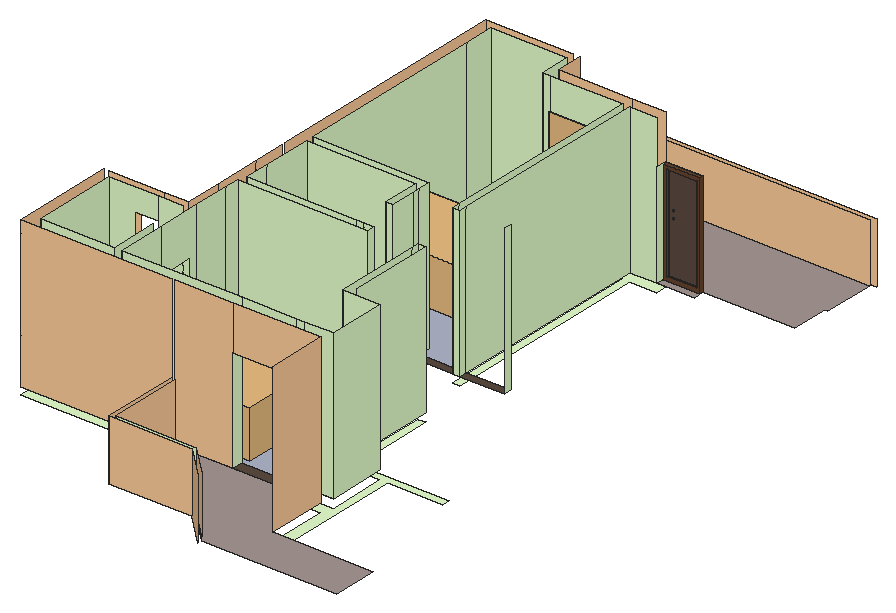
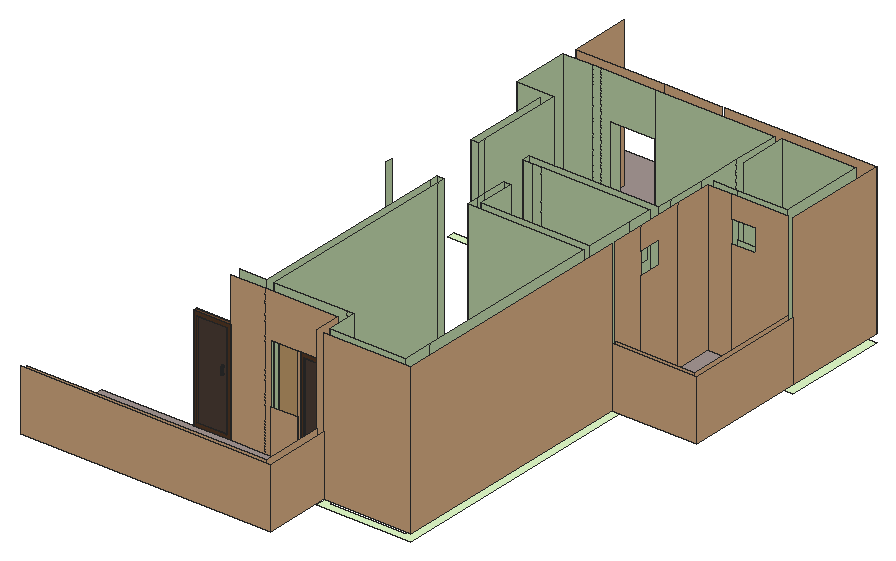
# SketchUp Ruby script. Lengths in inches.
U = 1.inch
M = Sketchup.active_model
def pt(a) = Geom::Point3d.new(a.map { |v| v * U })
def face(e, loops, mat)
  f = e.add_face(loops[0].map { |a| pt(a) })
  loops[1..].each { |l| e.add_face(l.map { |a| pt(a) }).erase! }
  f.material = f.back_material = mat if mat
  f
end
# faces: each face lists its corners as indices into pts; further lists are holes
def faces(e, pts, list, mat = nil) = list.each { |f| face(e, (f[0].is_a?(Array) ? f : [f]).map { |l| l.map { |i| pts[i] } }, mat) }
# xy, xz, yz: faces in a plane at the given z, y or x. An outline is a flat list of corners, or four numbers for a rectangle; further outlines are holes
def ring(l) = l.size == 4 ? [[l[0], l[1]], [l[2], l[1]], [l[2], l[3]], [l[0], l[3]]] : l.each_slice(2).to_a
def flat(e, list, mat, &to3) = list.each { |f| face(e, (f[0].is_a?(Array) ? f : [f]).map { |l| ring(l).map { |u, v| to3.(u, v) } }, mat) }
def xy(e, z, list, mat = nil) = flat(e, list, mat) { |x, y| [x, y, z] }
def xz(e, y, list, mat = nil) = flat(e, list, mat) { |x, z| [x, y, z] }
def yz(e, x, list, mat = nil) = flat(e, list, mat) { |y, z| [x, y, z] }
def lines(e, pts, list) = list.each { |a, b| e.add_line(pt(pts[a]), pt(pts[b])) }
# prism: a flat outline (further loops are holes) pulled along v
def prism(e, loops, v, mat = nil)
  f = face(e, loops, mat); d = Geom::Vector3d.new(v.map { |x| x * U })
  f.pushpull(f.normal.samedirection?(d) ? d.length : -d.length)
end
def box(e, o, s, mat = nil) = prism(e, [[o, [o[0] + s[0], o[1], o[2]], [o[0] + s[0], o[1] + s[1], o[2]], [o[0], o[1] + s[1], o[2]]]], [0, 0, s[2]], mat)
def at(x, y, z, deg = 0) = Geom::Transformation.translation(pt([x, y, z])) * Geom::Transformation.rotation(ORIGIN, Z_AXIS, deg.degrees)
def axes(o, x, y, z) = Geom::Transformation.new([*x, 0, *y, 0, *z, 0, *pt(o).to_a, 1])
def part(name) = M.definitions.add(name)
# library, detail: a bought-in or finely detailed component or shape, given as its bounding box
def library(name, o, s) = part(name).tap { |d| box(d.entities, o, s) }
def detail(e, o, s) = box(e.add_group.entities, o, s)
def put(e, d, t, mat = nil) = e.add_instance(d, t).tap { |i| i.material = mat if mat }
def group(e, t, mat = nil) = e.add_group.tap { |g| g.transformation = t; g.material = mat if mat }.entities
root = M.entities
M.materials.add("C02_Golden_Beige").color = [255, 205, 155]
M.materials.add("F01_Seafoam_Drift").color = [229, 255, 204]
M.materials.add("M01_Silver_Fog").color = [224, 224, 224]
M.materials.add("M03_Pewter_Shine").color = [168, 168, 168]
M.materials.add("M04_Stone_Frost").color = [142, 142, 142]
M.materials.add("M09_Shadow_Night").color = [0, 0, 0]
M.materials.add("Marble_03_1K").color = [175, 182, 201]
M.materials.add("Marble_06_1K").color = [165, 150, 147]
M.materials.add("Marble_20_1K").color = [172, 173, 182]
M.materials.add("Metal_06_1K").color = [238, 236, 231]
M.materials.add("Wood_Floor_12_1K").color = [92, 75, 65]
M.materials.add("Wood_Veneer_15_1K").color = [103, 69, 45]
c1 = library("Toilet 005",[-7.26,-21.97,0],[14.52,21.97,16.93])
c2 = library("Marcel Lift Bed Queen",[-31.83,-34.39,0],[63.66,83.19,38.98])
c3 = part("Group\#9")
xy(c3.entities,0,[[0,0,40.3125,19.1]])
xy(c3.entities,16,[[8.1875,0.77,29.4,18.21]])
xy(c3.entities,21.0625,[[0,0,40.3125,19.1]])
xy(c3.entities,25,[[[0,0,40.3125,19.1],[8.1875,0.77,29.4,18.21]]])
xy(c3.entities,25.5,[[[0,0,40.3125,19.1],[8.1875,0.77,29.4,18.21]]],"M09_Shadow_Night")
xz(c3.entities,-0.1875,[[20.17,22.3,20.39,22.33,20.61,22.42,20.79,22.56,20.93,22.74,21.01,22.95,21.04,23.18,21.01,23.4,20.93,23.61,20.79,23.8,20.61,23.93,20.39,24.02,20.17,24.05,19.94,24.02,19.73,23.93,19.55,23.8,19.41,23.61,19.32,23.4,19.29,23.18,19.32,22.95,19.41,22.74,19.55,22.56,19.73,22.42,19.94,22.33]],"M03_Pewter_Shine")
xz(c3.entities,0,[[19.56,0,20.76,21.0625],[0,25,40.3125,25.5]],"M09_Shadow_Night")
xz(c3.entities,0,[[0,0,19.56,21.0625],[20.76,0,40.3125,21.0625],[[0,21.0625,40.3125,25],[20.17,22.3,19.94,22.33,19.73,22.42,19.55,22.56,19.41,22.74,19.32,22.95,19.29,23.18,19.32,23.4,19.41,23.61,19.55,23.8,19.73,23.93,19.94,24.02,20.17,24.05,20.39,24.02,20.61,23.93,20.79,23.8,20.93,23.61,21.01,23.4,21.04,23.18,21.01,22.95,20.93,22.74,20.79,22.56,20.61,22.42,20.39,22.33]]],"Wood_Veneer_15_1K")
xz(c3.entities,0.77,[[8.1875,16,29.4,25]])
xz(c3.entities,0.77,[[8.1875,25,29.4,25.5]],"M04_Stone_Frost")
xz(c3.entities,18.21,[[8.1875,16,29.4,25],[8.1875,25,29.4,25.5]])
xz(c3.entities,19.1,[[0,25,40.3125,25.5]],"M09_Shadow_Night")
xz(c3.entities,19.1,[[0,0,40.3125,21.0625],[0,21.0625,40.3125,25]],"Wood_Veneer_15_1K")
yz(c3.entities,0,[[0,25,19.1,25.5]],"M09_Shadow_Night")
yz(c3.entities,0,[[0,0,19.1,21.0625],[0,21.0625,19.1,25]],"Wood_Veneer_15_1K")
yz(c3.entities,8.1875,[[0.77,16,18.21,25]])
yz(c3.entities,8.1875,[[0.77,25,18.21,25.5]],"M04_Stone_Frost")
yz(c3.entities,29.4,[[0.77,16,18.21,25]])
yz(c3.entities,29.4,[[0.77,25,18.21,25.5]],"M04_Stone_Frost")
yz(c3.entities,40.3125,[[0,25,19.1,25.5]],"M09_Shadow_Night")
yz(c3.entities,40.3125,[[0,0,19.1,21.0625],[0,21.0625,19.1,25]],"Wood_Veneer_15_1K")
p = [[19.73,0,22.42],[19.94,0,22.33],[19.94,-0.1875,22.33],[19.73,-0.1875,22.42],[20.17,0,22.3],[20.17,-0.1875,22.3],
  [20.39,0,22.33],[20.39,-0.1875,22.33],[20.61,0,22.42],[20.61,-0.1875,22.42],[19.55,0,22.56],[19.55,-0.1875,22.56],
  [20.79,0,22.56],[20.79,-0.1875,22.56],[19.41,0,22.74],[19.41,-0.1875,22.74],[20.93,0,22.74],[20.93,-0.1875,22.74],
  [19.32,0,22.95],[19.32,-0.1875,22.95],[21.01,0,22.95],[21.01,-0.1875,22.95],[19.29,0,23.18],[19.29,-0.1875,23.18],
  [21.04,0,23.18],[21.04,-0.1875,23.18],[19.32,0,23.4],[19.32,-0.1875,23.4],[21.01,0,23.4],[21.01,-0.1875,23.4],
  [19.41,0,23.61],[19.41,-0.1875,23.61],[20.93,0,23.61],[20.93,-0.1875,23.61],[19.55,0,23.8],[19.55,-0.1875,23.8],
  [20.79,0,23.8],[20.79,-0.1875,23.8],[19.73,0,23.93],[19.73,-0.1875,23.93],[20.61,0,23.93],[20.61,-0.1875,23.93],
  [19.94,0,24.02],[19.94,-0.1875,24.02],[20.39,0,24.02],[20.39,-0.1875,24.02],[20.17,0,24.05],[20.17,-0.1875,24.05]]
faces(c3.entities,p,[[0,1,2,3],[1,4,5,2],[4,6,7,5],[6,8,9,7],[10,0,3,11],[8,12,13,9],[14,10,11,15],[12,16,17,13],
  [18,14,15,19],[16,20,21,17],[22,18,19,23],[20,24,25,21],[26,22,23,27],[24,28,29,25],[30,26,27,31],[28,32,33,29],
  [34,30,31,35],[32,36,37,33],[38,34,35,39],[36,40,41,37],[42,38,39,43],[40,44,45,41],[46,42,43,47],[44,46,47,45]],"M03_Pewter_Shine")
g1 = group(c3.entities,at(16.89,0,11.23),"M01_Silver_Fog")
box(g1,[0,-0.1875,0],[1.125,0.1875,4],"M03_Pewter_Shine")
g2 = group(c3.entities,at(22.02,0,11.23),"M01_Silver_Fog")
box(g2,[0,-0.1875,0],[1.125,0.1875,4],"M03_Pewter_Shine")
c4 = part("Group\#25")
xy(c4.entities,0,[[0,-3,30,0]],"Wood_Veneer_15_1K")
xy(c4.entities,3,[[3,-2.25,27,0]],"Wood_Floor_12_1K")
xy(c4.entities,3,[[3,-3,27,-2.25]],"Wood_Veneer_15_1K")
xy(c4.entities,81,[[3,-2.25,27,0]],"Wood_Floor_12_1K")
xy(c4.entities,81,[[3,-3,27,-2.25]],"Wood_Veneer_15_1K")
xy(c4.entities,84,[[0,-3,30,0]],"Wood_Veneer_15_1K")
xz(c4.entities,-3,[[[0,0,30,84],[3,3,27,81]]],"Wood_Veneer_15_1K")
xz(c4.entities,-2.25,[[3,3,27,81]],"Wood_Floor_12_1K")
xz(c4.entities,0,[[[0,0,30,84],[3,3,27,81]]],"Wood_Veneer_15_1K")
yz(c4.entities,0,[[-3,0,0,84]],"Wood_Veneer_15_1K")
yz(c4.entities,3,[[-2.25,3,0,81]],"Wood_Floor_12_1K")
yz(c4.entities,3,[[-3,3,-2.25,81]],"Wood_Veneer_15_1K")
yz(c4.entities,27,[[-2.25,3,0,81]],"Wood_Floor_12_1K")
yz(c4.entities,27,[[-3,3,-2.25,81]],"Wood_Veneer_15_1K")
yz(c4.entities,30,[[-3,0,0,84]],"Wood_Veneer_15_1K")
g3 = group(c4.entities,at(22.875,-2.25,50.47),"Metal_06_1K")
xy(g3,-5.5625,[[0,-0.48,1.25,0]],"Metal_06_1K")
xy(g3,-4.9375,[[0,-1.375,1.25,-0.48]],"Metal_06_1K")
xy(g3,-4.6875,[[0,-1.125,1.25,0]],"Metal_06_1K")
xy(g3,-4.6875,[[0,-1.375,1.25,-1.125]],"Wood_Veneer_15_1K")
xy(g3,0,[[0,-1.125,1.25,-0.5],[0,-0.5,1.25,0]],"Metal_06_1K")
xy(g3,0.25,[[0,-1.375,1.25,-1.125],[0,-1.125,1.25,-0.5]],"Metal_06_1K")
xy(g3,0.25,[[0,-0.5,1.25,0]],"Wood_Veneer_15_1K")
xy(g3,1.25,[[0,-0.5,1.25,0]],"Metal_06_1K")
xz(g3,-1.375,[[0,-4.9375,1.25,-4.6875],[0,-4.6875,1.25,0.25]],"Metal_06_1K")
xz(g3,-1.125,[[0,-4.6875,1.25,0],[0,0,1.25,0.25]],"Metal_06_1K")
xz(g3,-0.5,[[0,0.25,1.25,1.25]],"Metal_06_1K")
xz(g3,-0.5,[[0,0,1.25,0.25]],"Wood_Veneer_15_1K")
xz(g3,-0.48,[[0,-5.5625,1.25,-4.9375]],"Metal_06_1K")
xz(g3,0,[[0,0.25,1.25,1.25]],"Metal_06_1K")
xz(g3,0,[[0,-5.5625,1.25,-4.6875],[0,0,1.25,0.25]],"Wood_Veneer_15_1K")
yz(g3,0,[[-0.48,-5.5625,-0.48,-4.9375,-1.375,-4.9375,-1.375,-4.6875,0,-4.6875,0,-5.5625],[-1.375,-4.6875,-1.125,0.25],[-1.125,0,-0.5,0.25],[-0.5,0,0,0.25],[-0.5,0.25,0,1.25]],"Metal_06_1K")
yz(g3,1.25,[[-0.48,-5.5625,0,-5.5625,0,-4.6875,-1.375,-4.6875,-1.375,-4.9375,-0.48,-4.9375],[-1.375,-4.6875,-1.125,0.25],[-1.125,0,-0.5,0.25],[-0.5,0,0,0.25],[-0.5,0.25,0,1.25]],"Metal_06_1K")
c5 = library("Group\#19",[0,0,0],[54,1.88,94.04])
xy(root,138.375,[[1619.1875,1117.375,1649.1875,1126.375]],"C02_Golden_Beige")
xy(root,142,[[1716.8125,714.6875,1767.92,714.6875,1767.92,723.6875,1725.8125,723.6875,1725.8125,819.6875,1770.625,819.6875,1770.625,825.6875,1695.8125,825.6875,1695.8125,895.375,1689.8125,895.375,1689.8125,819.6875,1719.8125,819.6875,1719.8125,772.375,1645.59,772.375,1645.59,763.375,1716.8125,763.375],[1473.8125,763.375,1645.59,763.375,1645.59,772.375,1548.8125,772.375,1548.8125,811.375,1542.8125,811.375,1542.8125,772.375,1482.8125,772.375,1482.8125,841.375,1523.47,841.375,1523.47,847.375,1473.8125,847.375],[1542.8125,811.375,1548.8125,811.375,1548.8125,847.375,1523.47,847.375,1523.47,841.375,1542.8125,841.375],[1542.8125,847.375,1548.8125,877.375],[1542.8125,877.375,1548.8125,877.375,1548.8125,889.375,1653.8125,889.375,1653.8125,895.375,1551.8125,895.375,1551.8125,915.375,1542.8125,915.375],
  [1542.8125,915.375,1551.8125,915.375,1551.8125,955.375,1639.8125,955.375,1639.8125,925.375,1645.8125,925.375,1645.8125,961.375,1551.8125,961.375,1551.8125,1141.375,1613.1875,1141.375,1613.1875,1117.375,1619.1875,1117.375,1619.1875,1147.375,1542.8125,1147.375],[1677.8125,945.6875,1683.8125,945.6875,1683.8125,1117.375,1705.83,1117.375,1705.83,1126.375,1619.1875,1126.375,1619.1875,1117.375,1677.8125,1117.375]],"F01_Seafoam_Drift")
xy(root,149,[[1548.8125,772.375,1689.8125,889.375],[1689.8125,772.375,1719.8125,819.6875],[1645.8125,951.6875,1677.8125,951.6875,1677.8125,1117.375,1551.8125,1117.375,1551.8125,961.375,1645.8125,961.375]],"Marble_03_1K")
xy(root,149,[[1688.52,678.6875,1797.92,678.6875,1797.92,714.6875,1716.8125,714.6875,1716.8125,763.375,1599.1,763.375,1599.1,703.375,1664.03,703.375],[1482.8125,772.375,1542.8125,841.375],[1477.8125,847.375,1542.8125,941.875],[1551.8125,1117.375,1613.1875,1141.375],[1705.83,1117.375,1735.83,1126.375],
  [1619.1875,1126.375,1809.8125,1126.375,1809.8125,1156.375,1812.8125,1156.375,1812.8125,1198.375,1619.1875,1198.375]],"Marble_06_1K")
xy(root,149,[[1551.8125,895.375,1639.8125,955.375]],"Marble_20_1K")
xy(root,149,[[1645.59,763.375,1681.59,772.375],[1542.8125,811.375,1548.8125,841.375],[1653.8125,889.375,1689.8125,895.375],[1639.8125,895.375,1645.8125,925.375],[1645.8125,945.6875,1677.8125,951.6875],
  [1683.8125,945.6875,1719.8125,951.6875],[1649.1875,1117.375,1651.0625,1126.375]],"Wood_Floor_12_1K")
xz(root,700.375,[[1596.1,148,1662.78,197]],"C02_Golden_Beige")
xz(root,703.375,[[1599.1,149,1664.03,197]],"F01_Seafoam_Drift")
xz(root,763.375,[[1473.8125,148,1596.1,269],[1599.1,149,1645.59,269],[1681.59,149,1716.8125,149,1716.8125,269,1645.59,269,1645.59,233,1681.59,233]],"C02_Golden_Beige")
xz(root,772.375,[[1482.8125,149,1542.8125,269],[1548.8125,149,1645.59,269],[1681.59,149,1681.59,233,1645.59,233,1645.59,269,1689.8125,269,1689.8125,149],[1689.8125,149,1695.8125,269],[1695.8125,149,1719.8125,269]],"F01_Seafoam_Drift")
xz(root,811.375,[[1542.8125,149,1548.8125,233]],"F01_Seafoam_Drift")
xz(root,819.6875,[[1689.8125,149,1719.8125,269]],"F01_Seafoam_Drift")
xz(root,841.375,[[1482.8125,149,1523.47,149,1523.47,233,1504.12,233,1504.12,251,1523.47,251,1523.47,269,1482.8125,269],[1523.47,149,1542.8125,269],[1542.8125,149,1548.8125,233]],"F01_Seafoam_Drift")
xz(root,847.375,[[1477.8125,149,1477.8125,269,1523.47,269,1523.47,251,1504.12,251,1504.12,233,1523.47,233,1523.47,149],[1523.47,149,1542.8125,269]],"C02_Golden_Beige")
xz(root,889.375,[[1548.8125,149,1653.8125,269]],"F01_Seafoam_Drift")
xz(root,895.375,[[1551.8125,149,1639.8125,269],[1639.8125,149,1645.8125,269],[1645.8125,149,1653.8125,269],[1689.8125,149,1695.8125,269]],"F01_Seafoam_Drift")
xz(root,925.375,[[1639.8125,149,1645.8125,269]],"F01_Seafoam_Drift")
xz(root,941.875,[[1477.8125,149,1542.8125,197]],"C02_Golden_Beige")
xz(root,944.875,[[1473.8125,148,1542.8125,197]],"C02_Golden_Beige")
xz(root,945.6875,[[1677.8125,149,1683.8125,269]],"F01_Seafoam_Drift")
xz(root,955.375,[[1551.8125,149,1639.8125,269]],"F01_Seafoam_Drift")
xz(root,961.375,[[1551.8125,149,1645.8125,269]],"F01_Seafoam_Drift")
xz(root,1117.375,[[1619.1875,138.375,1649.1875,149]],"C02_Golden_Beige")
xz(root,1117.375,[[1613.1875,149,1619.1875,269],[1673.1875,149,1677.8125,149,1677.8125,269,1619.1875,269,1619.1875,233,1673.1875,233],[1683.8125,149,1705.83,269]],"F01_Seafoam_Drift")
xz(root,1117.375,[[1649.1875,149,1651.0625,233],[1651.0625,149,1673.1875,185]],"Wood_Floor_12_1K")
xz(root,1126.375,[[1619.1875,138.375,1649.1875,149],[1673.1875,149,1673.1875,233,1619.1875,233,1619.1875,269,1677.8125,269,1677.8125,149],[1649.1875,149,1651.0625,233],[1651.0625,149,1673.1875,185],[1677.8125,149,1705.83,269]],"C02_Golden_Beige")
xz(root,1141.375,[[1551.8125,149,1613.1875,269]],"F01_Seafoam_Drift")
xz(root,1147.375,[[1542.8125,148,1613.1875,269]],"C02_Golden_Beige")
xz(root,1198.375,[[1619.1875,149,1812.8125,197]],"C02_Golden_Beige")
xz(root,1201.375,[[1613.1875,148,1815.8125,197]],"C02_Golden_Beige")
yz(root,1473.8125,[[763.375,148,847.375,269],[847.375,148,944.875,197]],"C02_Golden_Beige")
yz(root,1477.8125,[[847.375,149,941.875,197]],"C02_Golden_Beige")
yz(root,1482.8125,[[772.375,149,841.375,269]],"F01_Seafoam_Drift")
yz(root,1542.8125,[[944.875,148,1147.375,269],[847.375,149,877.375,269],[877.375,149,877.375,269,915.375,269,915.375,251,897.17,251,897.17,233,915.375,233,915.375,149],[915.375,149,941.875,269]],"C02_Golden_Beige")
yz(root,1542.8125,[[772.375,149,811.375,269]],"F01_Seafoam_Drift")
yz(root,1548.8125,[[772.375,149,811.375,269],[841.375,149,847.375,149,847.375,269,811.375,269,811.375,233,841.375,233],[847.375,149,877.375,269],[877.375,149,889.375,269]],"F01_Seafoam_Drift")
yz(root,1551.8125,[[895.375,149,915.375,149,915.375,233,897.17,233,897.17,251,915.375,251,915.375,269,895.375,269],[915.375,149,955.375,269],[961.375,149,1117.375,269],[1117.375,149,1141.375,269]],"F01_Seafoam_Drift")
yz(root,1596.1,[[700.375,148,763.375,197]],"C02_Golden_Beige")
yz(root,1599.1,[[703.375,149,763.375,197]],"C02_Golden_Beige")
yz(root,1613.1875,[[1147.375,148,1201.375,197]],"C02_Golden_Beige")
yz(root,1613.1875,[[1117.375,149,1141.375,269]],"F01_Seafoam_Drift")
yz(root,1619.1875,[[1126.375,149,1147.375,269],[1147.375,149,1198.375,197]],"C02_Golden_Beige")
yz(root,1619.1875,[[1117.375,138.375,1126.375,233]],"F01_Seafoam_Drift")
yz(root,1639.8125,[[925.375,149,955.375,269]],"F01_Seafoam_Drift")
yz(root,1645.59,[[763.375,149,772.375,233]],"F01_Seafoam_Drift")
yz(root,1645.8125,[[925.375,149,945.6875,269],[945.6875,149,951.6875,269],[951.6875,149,961.375,269]],"F01_Seafoam_Drift")
yz(root,1649.1875,[[1117.375,138.375,1126.375,149]],"C02_Golden_Beige")
yz(root,1649.1875,[[1117.375,149,1126.375,233]],"Wood_Floor_12_1K")
yz(root,1651.0625,[[1117.375,149,1126.375,185]],"Wood_Floor_12_1K")
yz(root,1653.8125,[[889.375,149,895.375,269]],"F01_Seafoam_Drift")
yz(root,1677.8125,[[945.6875,149,951.6875,269],[951.6875,149,1117.375,269]],"F01_Seafoam_Drift")
yz(root,1681.59,[[763.375,149,772.375,233]],"F01_Seafoam_Drift")
yz(root,1683.8125,[[945.6875,149,951.6875,269],[951.6875,149,1117.375,269]],"F01_Seafoam_Drift")
yz(root,1689.8125,[[819.6875,149,889.375,269],[889.375,149,895.375,269]],"F01_Seafoam_Drift")
yz(root,1695.8125,[[825.6875,149,895.375,269]],"F01_Seafoam_Drift")
yz(root,1705.83,[[1117.375,149,1126.375,233]],"F01_Seafoam_Drift")
yz(root,1716.8125,[[714.6875,149,763.375,269]],"C02_Golden_Beige")
yz(root,1719.8125,[[772.375,149,819.6875,269],[945.6875,149,951.6875,269]],"F01_Seafoam_Drift")
p = [[1662.78,700.375,148],[1687.27,675.6875,148],[1687.27,675.6875,197],[1662.78,700.375,197],[1688.52,678.6875,149],[1664.03,703.375,149],
  [1664.03,703.375,197],[1688.52,678.6875,197]]
faces(root,p,[[0,1,2,3],[4,5,6,7]],"C02_Golden_Beige")
put(root,c1,at(1483.51,804.98,149,90),"M01_Silver_Fog")
put(root,c1,at(1553.39,922.33,149,90),"M01_Silver_Fog")
put(root,c2,at(1603.75,1033.625,149,90),"C02_Golden_Beige")
put(root,c2,at(1616.68,826.18,149,180),"C02_Golden_Beige")
put(root,c3,at(1599.5,936.27,149),"C02_Golden_Beige")
put(root,c4,at(1649.1875,1123.375,149,-180),"C02_Golden_Beige")
put(root,c5,at(1619.1875,1116.34,149),"C02_Golden_Beige")
put(root,c4,at(1735.83,1123.375,149,-180),"C02_Golden_Beige")
